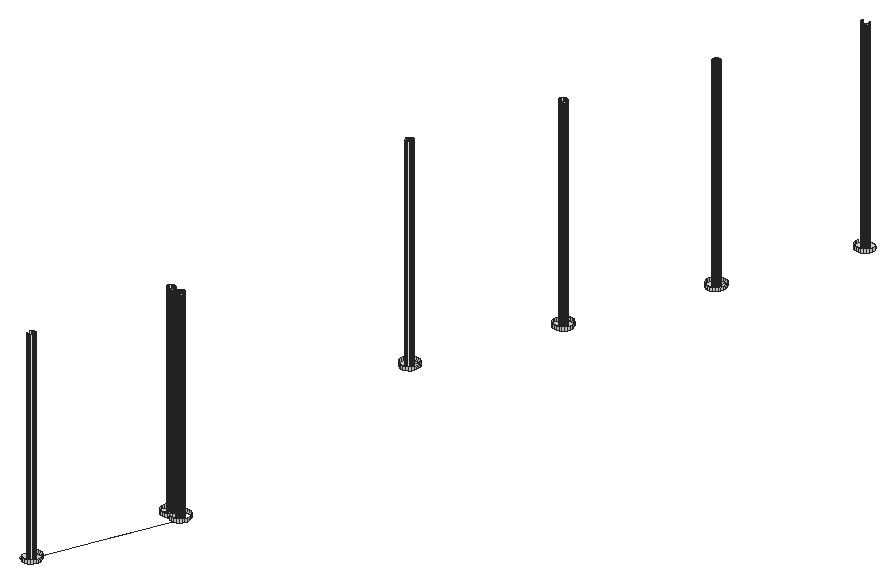
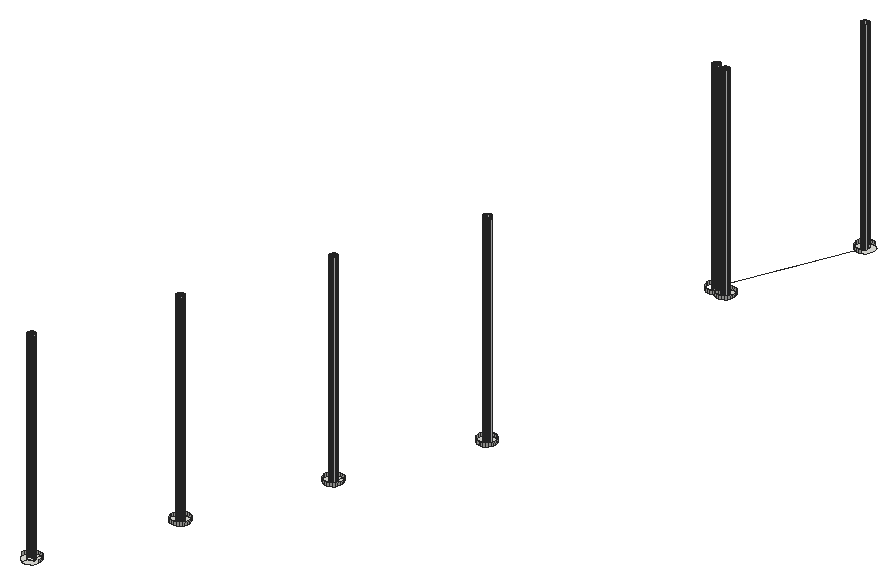
# SketchUp Ruby script. Lengths in inches.
U = 1.inch
M = Sketchup.active_model
def pt(a) = Geom::Point3d.new(a.map { |v| v * U })
def face(e, loops, mat)
  f = e.add_face(loops[0].map { |a| pt(a) })
  loops[1..].each { |l| e.add_face(l.map { |a| pt(a) }).erase! }
  f.material = f.back_material = mat if mat
  f
end
# faces: each face lists its corners as indices into pts; further lists are holes
def faces(e, pts, list, mat = nil) = list.each { |f| face(e, (f[0].is_a?(Array) ? f : [f]).map { |l| l.map { |i| pts[i] } }, mat) }
# xy, xz, yz: faces in a plane at the given z, y or x. An outline is a flat list of corners, or four numbers for a rectangle; further outlines are holes
def ring(l) = l.size == 4 ? [[l[0], l[1]], [l[2], l[1]], [l[2], l[3]], [l[0], l[3]]] : l.each_slice(2).to_a
def flat(e, list, mat, &to3) = list.each { |f| face(e, (f[0].is_a?(Array) ? f : [f]).map { |l| ring(l).map { |u, v| to3.(u, v) } }, mat) }
def xy(e, z, list, mat = nil) = flat(e, list, mat) { |x, y| [x, y, z] }
def xz(e, y, list, mat = nil) = flat(e, list, mat) { |x, z| [x, y, z] }
def yz(e, x, list, mat = nil) = flat(e, list, mat) { |y, z| [x, y, z] }
def lines(e, pts, list) = list.each { |a, b| e.add_line(pt(pts[a]), pt(pts[b])) }
# prism: a flat outline (further loops are holes) pulled along v
def prism(e, loops, v, mat = nil)
  f = face(e, loops, mat); d = Geom::Vector3d.new(v.map { |x| x * U })
  f.pushpull(f.normal.samedirection?(d) ? d.length : -d.length)
end
def box(e, o, s, mat = nil) = prism(e, [[o, [o[0] + s[0], o[1], o[2]], [o[0] + s[0], o[1] + s[1], o[2]], [o[0], o[1] + s[1], o[2]]]], [0, 0, s[2]], mat)
def at(x, y, z, deg = 0) = Geom::Transformation.translation(pt([x, y, z])) * Geom::Transformation.rotation(ORIGIN, Z_AXIS, deg.degrees)
def axes(o, x, y, z) = Geom::Transformation.new([*x, 0, *y, 0, *z, 0, *pt(o).to_a, 1])
def part(name) = M.definitions.add(name)
# library, detail: a bought-in or finely detailed component or shape, given as its bounding box
def library(name, o, s) = part(name).tap { |d| box(d.entities, o, s) }
def detail(e, o, s) = box(e.add_group.entities, o, s)
def put(e, d, t, mat = nil) = e.add_instance(d, t).tap { |i| i.material = mat if mat }
def group(e, t, mat = nil) = e.add_group.tap { |g| g.transformation = t; g.material = mat if mat }.entities
root = M.entities
M.materials.add("[Color_000]").color = [255, 255, 255]
xy(root,321.27,[[[973.7,833.66,974.1,833.74,974.47,833.93,974.78,834.2,975,834.54,975.13,834.93,975.16,835.34,975.08,835.75,974.89,836.11,974.62,836.42,974.28,836.65,974.21,836.67,973.89,836.78,973.48,836.8,973.07,836.72,972.7,836.53,972.4,836.26,972.17,835.92,972.04,835.53,972.02,835.12,972.1,834.72,972.28,834.35,972.56,834.04,972.9,833.8125,972.96,833.79,973.29,833.68],[973.63,834.6,973.47,834.61,973.34,834.66,973.3125,834.66,973.18,834.75,973.07,834.88,972.99,835.02,972.96,835.1875,972.97,835.35,973.02,835.51,973.11,835.64,973.23,835.75,973.38,835.83,973.54,835.86,973.71,835.85,973.84,835.81,973.86,835.8,974,835.71,974.11,835.58,974.18,835.4375,974.22,835.28,974.21,835.11,974.15,834.96,974.0625,834.82,973.94,834.71,973.79,834.64]],[973.3125,834.66,973.34,834.66,973.84,835.81,973.71,835.85,973.54,835.86,973.38,835.83,973.23,835.75,973.11,835.64,973.02,835.51,972.97,835.35,972.96,835.1875,972.99,835.02,973.07,834.88,973.18,834.75],[982.49,855.72,982.5,855.74,982.54,855.92,982.55,856.01,982.55,856.2,982.53,856.38,982.49,856.56,982.45,856.64,982.45,856.66,982.34,856.66,982.18,856.72,982.04,856.81,982,856.85,981.93,856.93,981.86,857.08,981.83,857.24,981.83,857.35,981.79,857.375,981.43,857.55,981.22,857.64,981.23,857.6,981.22,857.44,981.16,857.28,981.07,857.14,980.95,857.03,980.92,857.02,980.8,856.96,980.64,856.93,980.48,856.9375,980.32,856.99,980.18,857.08,980.08,857.2,980,857.35,979.97,857.51,979.98,857.67,980.03,857.83,980.12,857.97,980.24,858.07,979.33,858.46,979.18,858.24,979.05,857.85,979.03,857.44,979.11,857.04,979.29,856.67,979.57,856.36,979.91,856.14,980.3,856.01,980.71,855.98,981.11,856.07,981.34,856.18,981.42,856.09,981.77,855.87,982.16,855.74],[[980.71,855.98,981.11,856.07,981.34,856.18,981.48,856.25,981.79,856.52,982,856.85,981.93,856.93,981.86,857.08,981.83,857.24,981.83,857.35,981.87,857.33,981.95,857.28,982.02,857.23,982.09,857.17,982.11,857.15,982.14,857.26,982.17,857.67,982.09,858.07,981.9,858.4375,981.71,858.66,981.63,858.74,981.28,858.97,980.89,859.1,980.48,859.125,980.08,859.04,979.71,858.86,979.41,858.59,979.33,858.46,979.18,858.24,979.05,857.85,979.03,857.44,979.11,857.04,979.29,856.67,979.57,856.36,979.91,856.14,980.3,856.01],[980.64,856.93,980.48,856.9375,980.32,856.99,980.18,857.08,980.08,857.2,980,857.35,979.97,857.51,979.98,857.67,980.03,857.83,980.12,857.97,980.24,858.07,980.97,857.75,980.91,857.58,980.88,857.17,980.92,857.02,980.8,856.96],[981.22,857.64,980.97,857.75,981.04,857.97,981.05,857.99,981.12,857.91,981.19,857.76]],[982.34,856.66,982.18,856.72,982.04,856.81,982,856.85,982.01,856.87,982.11,857.15,982.22,857.04,982.28,856.96,982.33,856.89,982.42,856.73,982.45,856.66],
  [982,856.85,981.93,856.93,981.86,857.08,981.83,857.24,981.83,857.35,981.87,857.33,981.95,857.28,982.02,857.23,982.09,857.17,982.11,857.15,982.01,856.87],[980.64,856.93,980.8,856.96,980.92,857.02,980.88,857.17,980.91,857.58,980.97,857.75,980.24,858.07,980.12,857.97,980.03,857.83,979.98,857.67,979.97,857.51,980,857.35,980.08,857.2,980.18,857.08,980.32,856.99,980.48,856.9375],[980.92,857.02,980.88,857.17,980.91,857.58,980.97,857.75,981.22,857.64,981.23,857.6,981.22,857.44,981.16,857.28,981.07,857.14,980.95,857.03],[981.22,857.64,981.19,857.76,981.12,857.91,981.05,857.99,981.04,857.97,980.97,857.75],[[980.5,909.38,980.9,909.46,981.27,909.65,981.58,909.92,981.81,910.26,981.94,910.65,981.96,911.0625,981.88,911.47,981.69,911.83,981.42,912.14,981.08,912.37,981.01,912.39,980.6875,912.5,980.28,912.52,979.875,912.44,979.51,912.26,979.2,911.98,978.97,911.64,978.84,911.25,978.82,910.84,978.9,910.4375,979.08,910.07,979.36,909.76,979.7,909.54,979.76,909.51,980.09,909.41],[980.43,910.32,980.27,910.33,980.14,910.375,980.11,910.39,979.98,910.48,979.87,910.6,979.79,910.75,979.76,910.91,979.77,911.07,979.82,911.23,979.91,911.36,980.04,911.47,980.18,911.55,980.34,911.58,980.51,911.57,980.64,911.53,980.66,911.52,980.8,911.43,980.91,911.3,980.98,911.16,981.02,911,981.01,910.83,980.96,910.68,980.87,910.54,980.74,910.43,980.6,910.36]],
  [979.76,909.51,980.14,910.375,980.11,910.39,979.98,910.48,979.87,910.6,979.79,910.75,979.76,910.91,979.77,911.07,979.82,911.23,979.91,911.36,980.04,911.47,980.18,911.55,980.34,911.58,980.51,911.57,980.64,911.53,981.01,912.39,980.6875,912.5,980.28,912.52,979.875,912.44,979.51,912.26,979.2,911.98,978.97,911.64,978.84,911.25,978.82,910.84,978.9,910.4375,979.08,910.07,979.36,909.76,979.7,909.54],[980.14,910.375,980.64,911.53,980.51,911.57,980.34,911.58,980.18,911.55,980.04,911.47,979.91,911.36,979.82,911.23,979.77,911.07,979.76,910.91,979.79,910.75,979.87,910.6,979.98,910.48,980.11,910.39],[[990.14,931.52,990.55,931.6,990.91,931.79,991.22,932.0625,991.45,932.4,991.58,932.79,991.6,933.2,991.52,933.61,991.34,933.97,991.0625,934.28,990.72,934.51,990.33,934.64,989.92,934.66,989.52,934.58,989.15,934.4,988.84,934.12,988.62,933.78,988.49,933.39,988.46,932.98,988.54,932.58,988.73,932.21,989,931.9,989.34,931.68,989.41,931.65,989.73,931.55],[990.08,932.46,989.91,932.47,989.78,932.52,989.76,932.53,989.62,932.62,989.51,932.74,989.4375,932.89,989.4,933.05,989.41,933.21,989.46,933.37,989.56,933.5,989.68,933.61,989.83,933.6875,989.99,933.72,990.15,933.71,990.28,933.67,990.31,933.66,990.44,933.57,990.55,933.44,990.625,933.3,990.66,933.14,990.65,932.97,990.6,932.82,990.51,932.68,990.38,932.57,990.24,932.5]],[989.41,931.65,989.78,932.52,989.76,932.53,989.62,932.62,989.51,932.74,989.4375,932.89,989.4,933.05,989.41,933.21,989.46,933.37,989.56,933.5,989.68,933.61,989.83,933.6875,989.99,933.72,990.15,933.71,990.28,933.67,990.66,934.53,990.33,934.64,989.92,934.66,989.52,934.58,989.15,934.4,988.84,934.12,988.62,933.78,988.49,933.39,988.46,932.98,988.54,932.58,988.73,932.21,989,931.9,989.34,931.68],[989.78,932.52,990.28,933.67,990.15,933.71,989.99,933.72,989.83,933.6875,989.68,933.61,989.56,933.5,989.46,933.37,989.41,933.21,989.4,933.05,989.4375,932.89,989.51,932.74,989.62,932.62,989.76,932.53],
  [[999.76,953.6,1000.16,953.68,1000.53,953.87,1000.84,954.14,1001.07,954.49,1001.2,954.875,1001.22,955.29,1001.14,955.6875,1000.95,956.06,1000.68,956.36,1000.34,956.59,1000.27,956.61,999.95,956.72,999.54,956.74,999.13,956.66,998.77,956.48,998.46,956.2,998.23,955.86,998.1,955.47,998.08,955.06,998.16,954.66,998.34,954.29,998.62,953.98,998.96,953.76,999.02,953.74,999.35,953.625],[999.69,954.54,999.53,954.55,999.4,954.6,999.375,954.61,999.24,954.7,999.13,954.82,999.05,954.97,999.02,955.13,999.03,955.29,999.08,955.45,999.17,955.59,999.3,955.69,999.44,955.77,999.6,955.8,999.77,955.79,999.9,955.75,999.92,955.74,1000.0625,955.65,1000.17,955.53,1000.24,955.38,1000.28,955.22,1000.27,955.05,1000.22,954.9,1000.125,954.76,1000,954.65,999.85,954.58]],[999.02,953.74,999.4,954.6,999.375,954.61,999.24,954.7,999.13,954.82,999.05,954.97,999.02,955.13,999.03,955.29,999.08,955.45,999.17,955.59,999.3,955.69,999.44,955.77,999.6,955.8,999.77,955.79,999.9,955.75,1000.27,956.61,999.95,956.72,999.54,956.74,999.13,956.66,998.77,956.48,998.46,956.2,998.23,955.86,998.1,955.47,998.08,955.06,998.16,954.66,998.34,954.29,998.62,953.98,998.96,953.76],[999.4,954.6,999.9,955.75,999.77,955.79,999.6,955.8,999.44,955.77,999.3,955.69,999.17,955.59,999.08,955.45,999.03,955.29,999.02,955.13,999.05,954.97,999.13,954.82,999.24,954.7,999.375,954.61],[[1009.11,975.06,1009.51,975.14,1009.88,975.33,1010.18,975.6,1010.41,975.94,1010.54,976.33,1010.57,976.74,1010.48,977.15,1010.3,977.51,1010.03,977.82,1009.68,978.05,1009.29,978.18,1008.88,978.2,1008.48,978.12,1008.11,977.93,1007.8,977.66,1007.58,977.32,1007.45,976.93,1007.42,976.52,1007.51,976.12,1007.69,975.75,1007.96,975.44,1008.31,975.21,1008.7,975.08],[1009.04,976,1008.875,976.01,1008.74,976.06,1008.72,976.0625,1008.58,976.15,1008.47,976.28,1008.4,976.42,1008.37,976.59,1008.375,976.75,1008.43,976.91,1008.52,977.04,1008.64,977.15,1008.79,977.23,1008.95,977.26,1009.11,977.25,1009.24,977.21,1009.27,977.2,1009.41,977.11,1009.52,976.98,1009.59,976.84,1009.62,976.68,1009.61,976.51,1009.5625,976.36,1009.47,976.22,1009.35,976.11,1009.2,976.04]],[1008.37,975.19,1008.74,976.06,1008.72,976.0625,1008.58,976.15,1008.47,976.28,1008.4,976.42,1008.37,976.59,1008.375,976.75,1008.43,976.91,1008.52,977.04,1008.64,977.15,1008.79,977.23,1008.95,977.26,1009.11,977.25,1009.24,977.21,1009.62,978.07,1009.29,978.18,1008.88,978.2,1008.48,978.12,1008.11,977.93,1007.8,977.66,1007.58,977.32,1007.45,976.93,1007.42,976.52,1007.51,976.12,1007.69,975.75,1007.96,975.44,1008.31,975.21],
  [1008.74,976.06,1009.24,977.21,1009.11,977.25,1008.95,977.26,1008.79,977.23,1008.64,977.15,1008.52,977.04,1008.43,976.91,1008.375,976.75,1008.37,976.59,1008.4,976.42,1008.47,976.28,1008.58,976.15,1008.72,976.0625]])
xy(root,321.27,[[973.63,834.6,973.79,834.64,973.94,834.71,974.0625,834.82,974.15,834.96,974.21,835.11,974.22,835.28,974.18,835.4375,974.11,835.58,974,835.71,973.86,835.8,973.84,835.81,973.34,834.66,973.47,834.61],[982.5,856.65,982.66,856.6875,982.81,856.76,982.93,856.87,983.02,857.01,983.07,857.16,983.08,857.33,983.05,857.49,982.98,857.64,982.87,857.76,982.73,857.85,982.57,857.9,982.41,857.91,982.25,857.88,982.14,857.82,982.1,857.8,981.98,857.7,981.89,857.56,981.84,857.4,981.83,857.35,981.87,857.33,981.95,857.28,982.02,857.23,982.09,857.17,982.22,857.04,982.28,856.96,982.33,856.89,982.42,856.73,982.45,856.66],[980.97,857.75,981.04,857.97,981.05,857.99,981.01,858.03,980.87,858.12,980.72,858.17,980.55,858.18,980.39,858.15,980.24,858.08,980.24,858.07],[980.43,910.32,980.6,910.36,980.74,910.43,980.87,910.54,980.96,910.68,981.01,910.83,981.02,911,980.98,911.16,980.91,911.3,980.8,911.43,980.66,911.52,980.64,911.53,980.14,910.375,980.27,910.33],[990.08,932.46,990.24,932.5,990.38,932.57,990.51,932.68,990.6,932.82,990.65,932.97,990.66,933.14,990.625,933.3,990.55,933.44,990.44,933.57,990.31,933.66,990.28,933.67,989.78,932.52,989.91,932.47],
  [999.69,954.54,999.85,954.58,1000,954.65,1000.125,954.76,1000.22,954.9,1000.27,955.05,1000.28,955.22,1000.24,955.38,1000.17,955.53,1000.0625,955.65,999.92,955.74,999.9,955.75,999.4,954.6,999.53,954.55],[1009.04,976,1009.2,976.04,1009.35,976.11,1009.47,976.22,1009.5625,976.36,1009.61,976.51,1009.62,976.68,1009.59,976.84,1009.52,976.98,1009.41,977.11,1009.27,977.2,1009.24,977.21,1008.74,976.06,1008.875,976.01]],"[Color_000]")
p = [[972.9,833.8125,321.27],[972.96,833.79,321.27],[973.29,833.68,321.27],[973.29,833.68,321.86],[972.9,833.8125,321.86],[973.7,833.66,321.27],
  [973.7,833.66,321.86],[974.1,833.74,321.27],[974.1,833.74,321.86],[974.47,833.93,321.27],[974.47,833.93,321.86],[974.78,834.2,321.27],
  [974.78,834.2,321.86],[975,834.54,321.27],[975,834.54,321.86],[975.13,834.93,321.27],[975.13,834.93,321.86],[973.3125,834.66,321.27],
  [973.34,834.66,321.27],[973.47,834.61,321.27],[973.47,834.61,357.27],[973.3125,834.66,357.27],[973.63,834.6,321.27],[973.63,834.6,357.27],
  [973.79,834.64,321.27],[973.79,834.64,357.27],[973.94,834.71,321.27],[973.94,834.71,357.27],[973.18,834.75,321.27],[973.18,834.75,357.27],
  [974.0625,834.82,321.27],[974.0625,834.82,357.27],[973.07,834.88,321.27],[973.07,834.88,357.27],[974.15,834.96,321.27],[974.15,834.96,357.27],
  [975.16,835.34,321.27],[975.16,835.34,321.86],[974.21,835.11,321.27],[974.21,835.11,357.27],[974.22,835.28,321.27],[974.22,835.28,357.27],
  [974.18,835.4375,321.27],[974.18,835.4375,357.27],[975.08,835.75,321.27],[975.08,835.75,321.86],[974.11,835.58,321.27],[974.11,835.58,357.27],
  [973.11,835.64,321.27],[973.02,835.51,321.27],[973.02,835.51,357.27],[973.11,835.64,357.27],[973.23,835.75,321.27],[973.23,835.75,357.27],
  [974,835.71,321.27],[974,835.71,357.27],[973.86,835.8,321.27],[973.86,835.8,357.27],[974.89,836.11,321.27],[974.89,836.11,321.86],
  [973.38,835.83,321.27],[973.38,835.83,357.27],[973.54,835.86,321.27],[973.54,835.86,357.27],[973.71,835.85,321.27],[973.71,835.85,357.27],
  [973.84,835.81,321.27],[974.62,836.42,321.27],[974.62,836.42,321.86],[974.28,836.65,321.27],[974.28,836.65,321.86],[974.21,836.67,321.27],
  [973.89,836.78,321.27],[973.89,836.78,321.86],[973.48,836.8,321.27],[973.07,836.72,321.27],[973.07,836.72,321.86],[973.48,836.8,321.86],
  [981.77,855.87,321.27],[982.16,855.74,321.27],[982.16,855.74,321.86],[981.77,855.87,321.86],[982.49,855.72,321.27],[982.57,855.71,321.27],
  [982.57,855.71,321.86],[982.97,855.8,321.27],[982.97,855.8,321.86],[983.34,855.98,321.27],[983.34,855.98,321.86],[981.42,856.09,321.27],
  [981.42,856.09,321.86],[979.91,856.14,321.27],[980.3,856.01,321.27],[980.3,856.01,321.86],[979.91,856.14,321.86],[980.71,855.98,321.27],
  [980.71,855.98,321.86],[981.11,856.07,321.27],[981.11,856.07,321.86],[983.65,856.25,321.27],[983.65,856.25,321.86],[979.57,856.36,321.27],
  [979.57,856.36,321.86],[981.34,856.18,321.27],[981.48,856.25,321.27],[981.48,856.25,321.86],[981.34,856.18,321.86],[981.15,856.4,321.27],
  [981.15,856.4,321.86],[981.79,856.52,321.27],[981.79,856.52,321.86],[983.87,856.6,321.27],[983.87,856.6,321.86],[979.29,856.67,321.27],
  [979.29,856.67,321.86],[980.97,856.77,321.27],[980.97,856.77,321.86],[982,856.85,321.27],[982.01,856.87,321.27],[982.01,856.87,321.86],
  [984,856.99,321.27],[984,856.99,321.86],[979.11,857.04,321.27],[979.11,857.04,321.86],[982.04,856.81,321.27],[982.18,856.72,321.27],
  [982.18,856.72,357.27],[982.04,856.81,357.27],[982.34,856.66,321.27],[982.34,856.66,357.27],[982.45,856.66,321.27],[982.5,856.65,321.27],
  [982.5,856.65,357.27],[982.66,856.6875,321.27],[982.66,856.6875,357.27],[982.81,856.76,321.27],[982.81,856.76,357.27],[980.88,857.17,321.27],
  [980.92,857.02,321.27],[980.88,857.17,321.86],[981.93,856.93,321.27],[981.93,856.93,357.27],[982.93,856.87,321.27],[982.93,856.87,357.27],
  [980.32,856.99,321.27],[980.48,856.9375,321.27],[980.48,856.9375,357.27],[980.32,856.99,357.27],[980.64,856.93,321.27],[980.64,856.93,357.27],
  [980.8,856.96,321.27],[980.8,856.96,357.27],[981.86,857.08,321.27],[981.86,857.08,357.27],[982.11,857.15,321.27],[982.14,857.26,321.27],
  [982.14,857.26,321.86],[983.02,857.01,321.27],[983.02,857.01,357.27],[979.03,857.44,321.27],[979.03,857.44,321.86],[980.18,857.08,321.27],
  [980.18,857.08,357.27],[980.95,857.03,321.27],[980.95,857.03,357.27],[981.07,857.14,321.27],[981.07,857.14,357.27],[983.07,857.16,321.27],
  [983.07,857.16,357.27],[984.03,857.4,321.27],[984.03,857.4,321.86],[980.08,857.2,321.27],[980.08,857.2,357.27],[981.16,857.28,321.27],
  [981.16,857.28,357.27],[981.83,857.24,321.27],[981.83,857.24,357.27],[980,857.35,321.27],[980,857.35,357.27],[980.91,857.58,321.27],
  [980.91,857.58,321.86],[981.84,857.4,321.27],[981.83,857.35,321.27],[981.84,857.4,357.27],[983.08,857.33,321.27],[983.08,857.33,357.27],
  [979.97,857.51,321.27],[979.97,857.51,357.27],[981.22,857.44,321.27],[981.22,857.44,357.27],[982.17,857.67,321.27],[982.17,857.67,321.86],
  [983.05,857.49,321.27],[983.05,857.49,357.27],[979.05,857.85,321.27],[979.05,857.85,321.86],[981.23,857.6,321.27],[981.23,857.6,357.27],
  [981.89,857.56,321.27],[981.89,857.56,357.27],[983.94,857.8,321.27],[983.94,857.8,321.86],[979.98,857.67,321.27],[979.98,857.67,357.27],
  [982.98,857.64,321.27],[982.98,857.64,357.27],[981.04,857.97,321.27],[980.97,857.75,321.27],[981.04,857.97,321.86],[981.22,857.64,321.27],
  [981.19,857.76,321.27],[981.19,857.76,357.27],[981.98,857.7,321.27],[981.98,857.7,357.27],[982.87,857.76,321.27],[982.87,857.76,357.27],
  [980.03,857.83,321.27],[980.03,857.83,357.27],[982.1,857.8,321.27],[982.1,857.8,357.27],[982.14,857.82,321.27],[982.09,858.07,321.27],
  [982.09,858.07,321.86],[980.12,857.97,321.27],[980.12,857.97,357.27],[981.12,857.91,321.27],[981.12,857.91,357.27],[982.25,857.88,321.27],
  [982.25,857.88,357.27],[982.73,857.85,321.27],[982.57,857.9,321.27],[982.57,857.9,357.27],[982.73,857.85,357.27],[983.76,858.17,321.27],
  [983.76,858.17,321.86],[979.18,858.24,321.27],[979.18,858.24,321.86],[981.05,857.99,321.27],[981.01,858.03,321.27],[981.01,858.03,357.27],
  [982.41,857.91,321.27],[982.41,857.91,357.27],[980.24,858.08,321.27],[980.24,858.07,321.27],[980.24,858.08,357.27],[980.87,858.12,321.27],
  [980.87,858.12,357.27],[981.26,858.3125,321.27],[981.26,858.3125,321.86],[980.39,858.15,321.27],[980.39,858.15,357.27],[980.55,858.18,321.27],
  [980.55,858.18,357.27],[980.72,858.17,321.27],[980.72,858.17,357.27],[981.9,858.4375,321.27],[981.9,858.4375,321.86],[979.41,858.59,321.27],
  [979.33,858.46,321.27],[979.41,858.59,321.86],[983.49,858.47,321.27],[983.49,858.47,321.86],[981.57,858.59,321.27],[981.57,858.59,321.86],
  [981.71,858.66,321.27],[981.63,858.74,321.27],[981.63,858.74,321.86],[981.71,858.66,321.86],[983.14,858.7,321.27],[983.14,858.7,321.86],
  [979.71,858.86,321.27],[979.71,858.86,321.86],[981.94,858.77,321.27],[981.94,858.77,321.86],[981.28,858.97,321.27],[981.28,858.97,321.86],
  [982.75,858.83,321.27],[982.75,858.83,321.86],[982.34,858.85,321.27],[982.34,858.85,321.86],[980.08,859.04,321.27],[980.08,859.04,321.86],
  [980.48,859.125,321.27],[980.48,859.125,321.86],[980.89,859.1,321.27],[980.89,859.1,321.86],[979.7,909.54,321.27],[979.76,909.51,321.27],
  [980.09,909.41,321.27],[980.09,909.41,321.86],[979.7,909.54,321.86],[980.5,909.38,321.27],[980.5,909.38,321.86],[980.9,909.46,321.27],
  [980.9,909.46,321.86],[979.36,909.76,321.27],[979.36,909.76,321.86],[981.27,909.65,321.27],[981.27,909.65,321.86],[981.58,909.92,321.27],
  [981.58,909.92,321.86],[979.08,910.07,321.27],[979.08,910.07,321.86],[981.81,910.26,321.27],[981.81,910.26,321.86],[978.9,910.4375,321.27],
  [978.9,910.4375,321.86],[980.11,910.39,321.27],[980.14,910.375,321.27],[980.27,910.33,321.27],[980.27,910.33,357.27],[980.11,910.39,357.27],
  [980.43,910.32,321.27],[980.43,910.32,357.27],[980.6,910.36,321.27],[980.6,910.36,357.27],[981.94,910.65,321.27],[981.94,910.65,321.86],
  [978.82,910.84,321.27],[978.82,910.84,321.86],[979.98,910.48,321.27],[979.98,910.48,357.27],[980.74,910.43,321.27],[980.74,910.43,357.27],
  [980.87,910.54,321.27],[980.87,910.54,357.27],[979.87,910.6,321.27],[979.87,910.6,357.27],[980.96,910.68,321.27],[980.96,910.68,357.27],
  [979.79,910.75,321.27],[979.79,910.75,357.27],[979.76,910.91,321.27],[979.76,910.91,357.27],[981.01,910.83,321.27],[981.01,910.83,357.27],
  [981.96,911.0625,321.27],[981.96,911.0625,321.86],[978.84,911.25,321.27],[978.84,911.25,321.86],[981.02,911,321.27],[981.02,911,357.27],
  [979.77,911.07,321.27],[979.77,911.07,357.27],[980.98,911.16,321.27],[980.98,911.16,357.27],[979.82,911.23,321.27],[979.82,911.23,357.27],
  [981.88,911.47,321.27],[981.88,911.47,321.86],[978.97,911.64,321.27],[978.97,911.64,321.86],[979.91,911.36,321.27],[979.91,911.36,357.27],
  [980.91,911.3,321.27],[980.91,911.3,357.27],[980.8,911.43,321.27],[980.8,911.43,357.27],[980.04,911.47,321.27],[980.04,911.47,357.27],
  [980.66,911.52,321.27],[980.66,911.52,357.27],[980.18,911.55,321.27],[980.18,911.55,357.27],[980.34,911.58,321.27],[980.34,911.58,357.27],
  [980.64,911.53,321.27],[980.51,911.57,321.27],[980.51,911.57,357.27],[981.69,911.83,321.27],[981.69,911.83,321.86],[979.2,911.98,321.27],
  [979.2,911.98,321.86],[981.42,912.14,321.27],[981.42,912.14,321.86],[979.51,912.26,321.27],[979.51,912.26,321.86],[981.08,912.37,321.27],
  [981.08,912.37,321.86],[979.875,912.44,321.27],[979.875,912.44,321.86],[980.28,912.52,321.27],[980.28,912.52,321.86],[981.01,912.39,321.27],
  [980.6875,912.5,321.27],[980.6875,912.5,321.86],[989.34,931.68,321.27],[989.41,931.65,321.27],[989.73,931.55,321.27],[989.73,931.55,321.86],
  [989.34,931.68,321.86],[990.14,931.52,321.27],[990.14,931.52,321.86],[990.55,931.6,321.27],[990.55,931.6,321.86],[990.91,931.79,321.27],
  [990.91,931.79,321.86],[989,931.9,321.27],[989,931.9,321.86],[991.22,932.0625,321.27],[991.22,932.0625,321.86],[988.73,932.21,321.27],
  [988.73,932.21,321.86],[991.45,932.4,321.27],[991.45,932.4,321.86],[988.54,932.58,321.27],[988.54,932.58,321.86],[991.58,932.79,321.27],
  [991.58,932.79,321.86],[989.62,932.62,321.27],[989.76,932.53,321.27],[989.76,932.53,357.27],[989.62,932.62,357.27],[989.78,932.52,321.27],
  [989.91,932.47,321.27],[989.91,932.47,357.27],[990.08,932.46,321.27],[990.08,932.46,357.27],[990.24,932.5,321.27],[990.24,932.5,357.27],
  [990.38,932.57,321.27],[990.38,932.57,357.27],[988.46,932.98,321.27],[988.46,932.98,321.86],[989.51,932.74,321.27],[989.51,932.74,357.27],
  [990.51,932.68,321.27],[990.51,932.68,357.27],[989.4375,932.89,321.27],[989.4375,932.89,357.27],[990.6,932.82,321.27],[990.6,932.82,357.27],
  [990.65,932.97,321.27],[990.65,932.97,357.27],[991.6,933.2,321.27],[991.6,933.2,321.86],[989.4,933.05,321.27],[989.4,933.05,357.27],
  [988.49,933.39,321.27],[988.49,933.39,321.86],[989.41,933.21,321.27],[989.41,933.21,357.27],[990.66,933.14,321.27],[990.66,933.14,357.27],
  [990.625,933.3,321.27],[990.625,933.3,357.27],[989.46,933.37,321.27],[989.46,933.37,357.27],[991.52,933.61,321.27],[991.52,933.61,321.86],
  [990.55,933.44,321.27],[990.55,933.44,357.27],[988.62,933.78,321.27],[988.62,933.78,321.86],[989.56,933.5,321.27],[989.56,933.5,357.27],
  [990.44,933.57,321.27],[990.44,933.57,357.27],[989.68,933.61,321.27],[989.68,933.61,357.27],[989.83,933.6875,321.27],[989.83,933.6875,357.27],
  [990.31,933.66,321.27],[990.31,933.66,357.27],[991.34,933.97,321.27],[991.34,933.97,321.86],[989.99,933.72,321.27],[989.99,933.72,357.27],
  [990.15,933.71,321.27],[990.15,933.71,357.27],[990.28,933.67,321.27],[988.84,934.12,321.27],[988.84,934.12,321.86],[991.0625,934.28,321.27],
  [991.0625,934.28,321.86],[989.15,934.4,321.27],[989.15,934.4,321.86],[990.72,934.51,321.27],[990.72,934.51,321.86],[989.52,934.58,321.27],
  [989.52,934.58,321.86],[990.66,934.53,321.27],[990.33,934.64,321.27],[990.33,934.64,321.86],[989.92,934.66,321.27],[989.92,934.66,321.86],
  [998.96,953.76,321.27],[999.02,953.74,321.27],[999.35,953.625,321.27],[999.35,953.625,321.86],[998.96,953.76,321.86],[999.76,953.6,321.27],
  [999.76,953.6,321.86],[1000.16,953.68,321.27],[1000.16,953.68,321.86],[1000.53,953.87,321.27],[1000.53,953.87,321.86],[998.62,953.98,321.27],
  [998.62,953.98,321.86],[1000.84,954.14,321.27],[1000.84,954.14,321.86],[998.34,954.29,321.27],[998.34,954.29,321.86],[1001.07,954.49,321.27],
  [1001.07,954.49,321.86],[998.16,954.66,321.27],[998.16,954.66,321.86],[999.53,954.55,321.27],[999.69,954.54,321.27],[999.69,954.54,357.27],
  [999.53,954.55,357.27],[999.85,954.58,321.27],[999.85,954.58,357.27],[1001.2,954.875,321.27],[1001.2,954.875,321.86],[999.24,954.7,321.27],
  [999.375,954.61,321.27],[999.375,954.61,357.27],[999.24,954.7,357.27],[999.4,954.6,321.27],[1000,954.65,321.27],[1000,954.65,357.27],
  [998.08,955.06,321.27],[998.08,955.06,321.86],[999.13,954.82,321.27],[999.13,954.82,357.27],[1000.125,954.76,321.27],[1000.125,954.76,357.27],
  [999.05,954.97,321.27],[999.05,954.97,357.27],[1000.22,954.9,321.27],[1000.22,954.9,357.27],[1000.27,955.05,321.27],[1000.27,955.05,357.27],
  [1001.22,955.29,321.27],[1001.22,955.29,321.86],[999.02,955.13,321.27],[999.02,955.13,357.27],[998.1,955.47,321.27],[998.1,955.47,321.86],
  [999.03,955.29,321.27],[999.03,955.29,357.27],[1000.28,955.22,321.27],[1000.28,955.22,357.27],[1000.24,955.38,321.27],[1000.24,955.38,357.27],
  [999.08,955.45,321.27],[999.08,955.45,357.27],[1001.14,955.6875,321.27],[1001.14,955.6875,321.86],[999.17,955.59,321.27],[999.17,955.59,357.27],
  [1000.17,955.53,321.27],[1000.17,955.53,357.27],[998.23,955.86,321.27],[998.23,955.86,321.86],[1000.0625,955.65,321.27],[1000.0625,955.65,357.27],
  [999.3,955.69,321.27],[999.3,955.69,357.27],[999.92,955.74,321.27],[999.92,955.74,357.27],[999.44,955.77,321.27],[999.44,955.77,357.27],
  [999.9,955.75,321.27],[999.77,955.79,321.27],[999.77,955.79,357.27],[1000.95,956.06,321.27],[1000.95,956.06,321.86],[999.6,955.8,321.27],
  [999.6,955.8,357.27],[998.46,956.2,321.27],[998.46,956.2,321.86],[1000.68,956.36,321.27],[1000.68,956.36,321.86],[998.77,956.48,321.27],
  [998.77,956.48,321.86],[1000.34,956.59,321.27],[1000.34,956.59,321.86],[999.13,956.66,321.27],[999.13,956.66,321.86],[1000.27,956.61,321.27],
  [999.95,956.72,321.27],[999.95,956.72,321.86],[999.54,956.74,321.27],[999.54,956.74,321.86],[1008.31,975.21,321.27],[1008.37,975.19,321.27],
  [1008.7,975.08,321.27],[1008.7,975.08,321.86],[1008.31,975.21,321.86],[1009.11,975.06,321.27],[1009.11,975.06,321.86],[1009.51,975.14,321.27],
  [1009.51,975.14,321.86],[1009.88,975.33,321.27],[1009.88,975.33,321.86],[1007.96,975.44,321.27],[1007.96,975.44,321.86],[1010.18,975.6,321.27],
  [1010.18,975.6,321.86],[1007.69,975.75,321.27],[1007.69,975.75,321.86],[1010.41,975.94,321.27],[1010.41,975.94,321.86],[1007.51,976.12,321.27],
  [1007.51,976.12,321.86],[1010.54,976.33,321.27],[1010.54,976.33,321.86],[1008.72,976.0625,321.27],[1008.74,976.06,321.27],[1008.875,976.01,321.27],
  [1008.875,976.01,357.27],[1008.72,976.0625,357.27],[1009.04,976,321.27],[1009.04,976,357.27],[1009.2,976.04,321.27],[1009.2,976.04,357.27],
  [1009.35,976.11,321.27],[1009.35,976.11,357.27],[1007.42,976.52,321.27],[1007.42,976.52,321.86],[1008.58,976.15,321.27],[1008.58,976.15,357.27],
  [1009.47,976.22,321.27],[1009.47,976.22,357.27],[1008.47,976.28,321.27],[1008.47,976.28,357.27],[1009.5625,976.36,321.27],[1009.5625,976.36,357.27],
  [1008.4,976.42,321.27],[1008.4,976.42,357.27],[1010.57,976.74,321.27],[1010.57,976.74,321.86],[1008.37,976.59,321.27],[1008.37,976.59,357.27],
  [1009.61,976.51,321.27],[1009.61,976.51,357.27],[1007.45,976.93,321.27],[1007.45,976.93,321.86],[1009.62,976.68,321.27],[1009.62,976.68,357.27],
  [1008.375,976.75,321.27],[1008.375,976.75,357.27],[1009.59,976.84,321.27],[1009.59,976.84,357.27],[1008.43,976.91,321.27],[1008.43,976.91,357.27],
  [1009.52,976.98,321.27],[1009.52,976.98,357.27],[982.32,855.29,321.27],[982.47,855.66,321.27]]
faces(root,p,[[0,1,2,3,4],[2,5,6,3],[5,7,8,6],[7,9,10,8],[9,11,12,10],[11,13,14,12],[13,15,16,14],[15,36,37,16],
  [36,44,45,37],[44,58,59,45],[58,67,68,59],[67,69,70,68],[69,71,72,73,70],[74,75,76,77],[72,74,77,73],[78,79,80,81],
  [79,82,83,84,80],[83,85,86,84],[85,87,88,86],[89,78,81,90],[91,92,93,94],[92,95,96,93],[95,97,98,96],[87,99,100,88],
  [101,91,94,102],[97,103,104,105,106,98],[107,103,89,90,106,108],[104,109,110,105],[99,111,112,100],[113,101,102,114],[115,107,108,116],[109,117,118,119,110],
  [111,120,121,112],[122,113,114,123],[137,138,115,116,139],[118,154,155,156,119],[159,122,123,160],[120,169,170,121],[179,137,139,180],[155,190,191,156],
  [194,159,160,195],[169,200,201,170],[206,207,179,180,208],[190,220,221,222,191],[200,233,234,201],[235,194,195,236],[247,237,206,208,248],[221,255,256,222],
  [257,258,235,236,259],[233,260,261,234],[262,247,248,263],[255,264,265,266,267,256],[260,268,269,261],[270,257,259,271],[272,264,262,263,267,273],[265,274,275,266],
  [268,276,277,269],[278,272,273,279],[276,278,279,277],[280,270,271,281],[282,280,281,283],[274,284,285,275],[284,282,283,285],[286,287,288,289,290],
  [288,291,292,289],[291,293,294,292],[295,286,290,296],[293,297,298,294],[297,299,300,298],[301,295,296,302],[299,303,304,300],[305,301,302,306],
  [303,316,317,304],[318,305,306,319],[316,336,337,317],[338,318,319,339],[336,348,349,337],[350,338,339,351],[348,369,370,349],[371,350,351,372],
  [369,373,374,370],[375,371,372,376],[373,377,378,374],[379,375,376,380],[381,379,380,382],[377,383,384,385,378],[384,381,382,385],[386,387,388,389,390],
  [388,391,392,389],[391,393,394,392],[393,395,396,394],[397,386,390,398],[395,399,400,396],[401,397,398,402],[399,403,404,400],[405,401,402,406],
  [403,407,408,404],[422,405,406,423],[407,434,435,408],[438,422,423,439],[434,448,449,435],[452,438,439,453],[448,464,465,449],[471,452,453,472],
  [464,473,474,465],[475,471,472,476],[473,477,478,474],[479,475,476,480],[477,481,482,483,478],[484,479,480,485],[482,484,485,483],[486,487,488,489,490],
  [488,491,492,489],[491,493,494,492],[493,495,496,494],[497,486,490,498],[495,499,500,496],[501,497,498,502],[499,503,504,500],[505,501,502,506],
  [503,513,514,504],[522,505,506,523],[513,534,535,514],[538,522,523,539],[534,548,549,535],[554,538,539,555],[548,567,568,549],[571,554,555,572],
  [567,573,574,568],[575,571,572,576],[573,577,578,574],[579,575,576,580],[577,581,582,583,578],[584,579,580,585],[582,584,585,583],[586,587,588,589,590],
  [588,591,592,589],[591,593,594,592],[593,595,596,594],[597,586,590,598],[595,599,600,596],[601,597,598,602],[599,603,604,600],[605,601,602,606],
  [603,607,608,604],[620,605,606,621],[607,632,633,608],[638,620,621,639]])
faces(root,p,[[17,18,19,20,21],[19,22,23,20],[22,24,25,23],[24,26,27,25],[28,17,21,29],[26,30,31,27],[32,28,29,33],[30,34,35,31],
  [34,38,39,35],[38,40,41,39],[40,42,43,41],[42,46,47,43],[48,49,50,51],[52,48,51,53],[46,54,55,47],[54,56,57,55],
  [60,52,53,61],[62,60,61,63],[64,62,63,65],[56,66,64,65,57],[124,125,126,127],[125,128,129,126],[128,130,131,132,129],[131,133,134,132],
  [133,135,136,134],[140,117,124,127,141],[135,142,143,136],[144,145,146,147],[145,148,149,146],[148,150,151,149],[152,140,141,153],[142,157,158,143],
  [161,144,147,162],[150,138,163,164,151],[163,165,166,164],[157,167,168,158],[171,161,162,172],[165,173,174,166],[175,152,153,176],[177,171,172,178],
  [181,182,175,176,183],[167,184,185,168],[186,177,178,187],[173,188,189,174],[184,192,193,185],[188,196,197,189],[198,181,183,199],[202,186,187,203],
  [192,204,205,193],[196,209,210,211,197],[212,198,199,213],[204,214,215,205],[216,202,203,217],[218,212,213,219],[223,216,217,224],[210,225,226,211],
  [227,220,218,219,228],[229,230,231,232],[214,229,232,215],[225,237,238,239,226],[240,227,228,241],[230,240,241,231],[242,243,223,224,244],[238,245,246,239],
  [249,242,244,250],[251,249,250,252],[245,253,254,246],[253,251,252,254],[307,308,309,310,311],[309,312,313,310],[312,314,315,313],[320,307,311,321],
  [314,322,323,315],[322,324,325,323],[326,320,321,327],[324,328,329,325],[330,326,327,331],[332,330,331,333],[328,334,335,329],[334,340,341,335],
  [342,332,333,343],[340,344,345,341],[346,342,343,347],[352,346,347,353],[344,354,355,345],[354,356,357,355],[358,352,353,359],[356,360,361,357],
  [362,358,359,363],[364,362,363,365],[360,366,367,368,361],[367,364,365,368],[409,410,411,412],[410,413,414,415,411],[414,416,417,415],[416,418,419,417],
  [418,420,421,419],[424,409,412,425],[420,426,427,421],[428,424,425,429],[426,430,431,427],[430,432,433,431],[436,428,429,437],[440,436,437,441],
  [432,442,443,433],[442,444,445,443],[446,440,441,447],[444,450,451,445],[454,446,447,455],[450,456,457,451],[458,454,455,459],[460,458,459,461],
  [456,462,463,457],[466,460,461,467],[468,466,467,469],[462,470,468,469,463],[507,508,509,510],[508,511,512,509],[515,516,517,518],[516,519,507,510,517],
  [511,520,521,512],[524,515,518,525],[520,526,527,521],[528,524,525,529],[526,530,531,527],[530,532,533,531],[536,528,529,537],[540,536,537,541],
  [532,542,543,533],[542,544,545,543],[546,540,541,547],[550,546,547,551],[544,552,553,545],[552,556,557,553],[558,550,551,559],[556,560,561,557],
  [562,558,559,563],[560,564,565,566,561],[569,562,563,570],[565,569,570,566],[609,610,611,612,613],[611,614,615,612],[614,616,617,615],[616,618,619,617],
  [622,609,613,623],[618,624,625,619],[626,622,623,627],[624,628,629,625],[630,626,627,631],[634,630,631,635],[628,636,637,629],[636,640,641,637],
  [642,634,635,643],[640,644,645,641],[646,642,643,647],[644,648,649,645]],"[Color_000]")
lines(root,p,[[650,651],[651,82],[71,650]])
